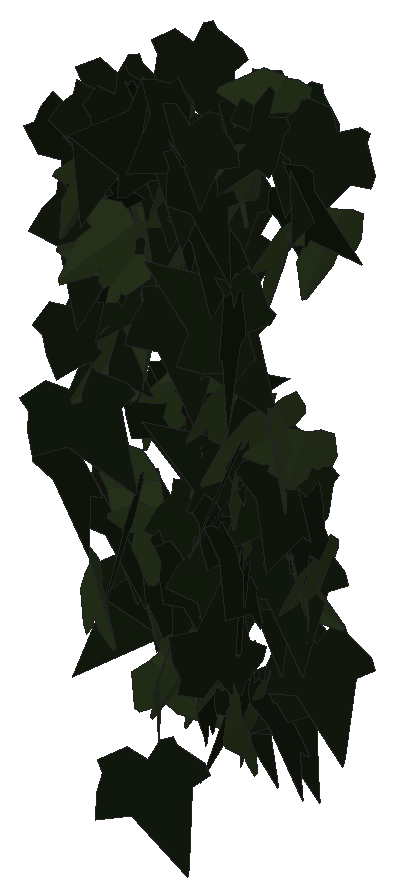
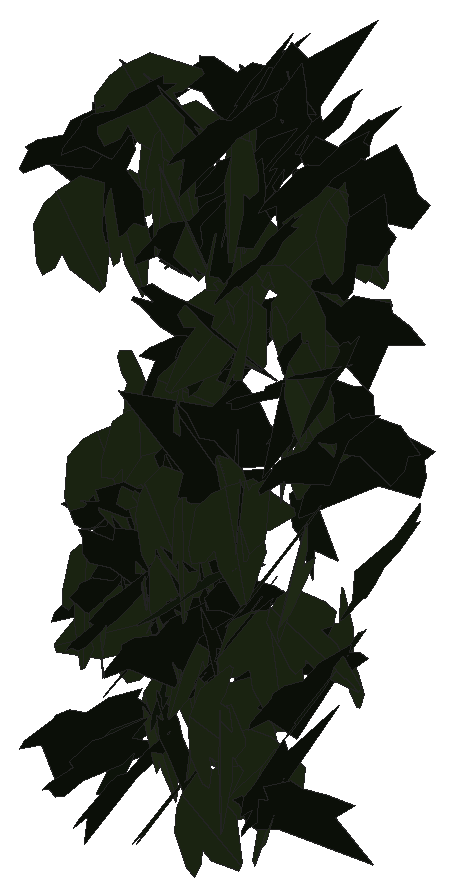
# SketchUp Ruby script. Lengths in inches.
U = 1.inch
M = Sketchup.active_model
def pt(a) = Geom::Point3d.new(a.map { |v| v * U })
def face(e, loops, mat)
  f = e.add_face(loops[0].map { |a| pt(a) })
  loops[1..].each { |l| e.add_face(l.map { |a| pt(a) }).erase! }
  f.material = f.back_material = mat if mat
  f
end
# faces: each face lists its corners as indices into pts; further lists are holes
def faces(e, pts, list, mat = nil) = list.each { |f| face(e, (f[0].is_a?(Array) ? f : [f]).map { |l| l.map { |i| pts[i] } }, mat) }
# xy, xz, yz: faces in a plane at the given z, y or x. An outline is a flat list of corners, or four numbers for a rectangle; further outlines are holes
def ring(l) = l.size == 4 ? [[l[0], l[1]], [l[2], l[1]], [l[2], l[3]], [l[0], l[3]]] : l.each_slice(2).to_a
def flat(e, list, mat, &to3) = list.each { |f| face(e, (f[0].is_a?(Array) ? f : [f]).map { |l| ring(l).map { |u, v| to3.(u, v) } }, mat) }
def xy(e, z, list, mat = nil) = flat(e, list, mat) { |x, y| [x, y, z] }
def xz(e, y, list, mat = nil) = flat(e, list, mat) { |x, z| [x, y, z] }
def yz(e, x, list, mat = nil) = flat(e, list, mat) { |y, z| [x, y, z] }
def lines(e, pts, list) = list.each { |a, b| e.add_line(pt(pts[a]), pt(pts[b])) }
# prism: a flat outline (further loops are holes) pulled along v
def prism(e, loops, v, mat = nil)
  f = face(e, loops, mat); d = Geom::Vector3d.new(v.map { |x| x * U })
  f.pushpull(f.normal.samedirection?(d) ? d.length : -d.length)
end
def box(e, o, s, mat = nil) = prism(e, [[o, [o[0] + s[0], o[1], o[2]], [o[0] + s[0], o[1] + s[1], o[2]], [o[0], o[1] + s[1], o[2]]]], [0, 0, s[2]], mat)
def at(x, y, z, deg = 0) = Geom::Transformation.translation(pt([x, y, z])) * Geom::Transformation.rotation(ORIGIN, Z_AXIS, deg.degrees)
def axes(o, x, y, z) = Geom::Transformation.new([*x, 0, *y, 0, *z, 0, *pt(o).to_a, 1])
def part(name) = M.definitions.add(name)
# library, detail: a bought-in or finely detailed component or shape, given as its bounding box
def library(name, o, s) = part(name).tap { |d| box(d.entities, o, s) }
def detail(e, o, s) = box(e.add_group.entities, o, s)
def put(e, d, t, mat = nil) = e.add_instance(d, t).tap { |i| i.material = mat if mat }
def group(e, t, mat = nil) = e.add_group.tap { |g| g.transformation = t; g.material = mat if mat }.entities
root = M.entities
M.materials.add("efeu1").color = [18, 25, 13]
M.materials.add("efeu2").color = [43, 57, 29]
c1 = part("ivyleaf_9")
p = [[1.54,2.16,1.25],[1.36,2.04,1.19],[-0.21,0.99,0.68],[-0.71,1.11,0.82],[-0.85,0.86,0.67],[-0.8,0.17,0.21],
  [-0.9,-0.01,0.1],[-0.67,-0.16,-0.02],[-0.08,-0.08,-0.05],[-0.03,-0.6,-0.4],[0.65,-0.88,-0.66],[0.83,-0.6,-0.49],
  [1.29,-0.42,-0.43],[1.8125,-0.07,-0.26],[1.21,0.44,0.15]]
faces(c1.entities,p,[[0,1,2,3,4,5,6,7,8,9,10,11,12,13,14]],"efeu1")
c2 = part("ivyleaf_10")
p = [[0,0.5,-0.03],[-0.0625,2.02,-0.43],[-0.19,2.01,-0.46],[-0.54,1.05,-0.29],[-0.52,0.625,-0.18],[-0.83,0.76,-0.28],
  [-1.16,0.64,-0.33],[-1.15,0.33,-0.24],[-0.77,-0.39,0.02],[-0.3,-0.51,0.16],[0.04,-0.48,0.23],[-0.02,2.01,-0.4375],
  [-0.06,2.01,-0.43],[0.04,-0.49,0.23],[0.67,-0.49,0.14],[1.38,0.36,-0.2],[1.375,0.51,-0.24],[0.81,0.65,-0.19],
  [0.62,0.59,-0.15],[0.6,1.09,-0.28],[0.5,1.23,-0.31]]
faces(c2.entities,p,[[0,1,2,3,4,5,6,7,8,9,10],[11,12,0,13,14,15,16,17,18,19,20]],"efeu2")
put(root,c1,axes([30.3,219.35,234.05],[-0.08289,-0.36968,-0.32629],[0.0657,0.31963,-0.37884],[0.48868,-0.10568,-0.00441]))
put(root,c2,axes([29.49,220.625,234.35],[0.06504,-0.16772,-0.46652],[0.15197,-0.44112,0.17978],[-0.47189,-0.16518,-0.00641]))
put(root,c1,axes([30.59,220.63,239.86],[-0.209,0.00128,-0.45422],[0.44781,-0.08313,-0.20629],[-0.07605,-0.49304,0.03361]))
put(root,c1,axes([29.08,220.65,236.79],[-0.26517,0.09797,-0.41242],[0.36855,-0.18705,-0.2814],[-0.20942,-0.45323,0.02698]))
put(root,c1,axes([30.46,220.92,236.13],[-0.00947,-0.27867,0.41503],[0.08144,-0.41042,-0.27372],[0.49323,0.06242,0.05316]))
put(root,c2,axes([30.86,220.47,234.28],[-0.27139,0.1393,0.39616],[-0.37466,0.13274,-0.30333],[-0.18968,-0.46149,0.03233]))
put(root,c1,axes([29.02,221,241.49],[-0.03894,-0.04823,0.49614],[-0.31224,-0.38557,-0.06199],[0.38857,-0.31466,-0.00009]))
put(root,c2,axes([28.22,220.84,235.23],[0.15955,-0.10346,0.46243],[0.43514,-0.16118,-0.1862],[0.1876,0.46186,0.03861]))
put(root,c1,axes([30.46,220.5,234.86],[-0.22152,-0.24857,0.37302],[0.25211,0.27495,0.33293],[-0.37064,0.33558,0.00352]))
put(root,c1,axes([30.5,220.85,235.49],[-0.07678,0.22238,0.44119],[0.04162,-0.44199,0.23003],[0.49231,0.07204,0.04936]))
put(root,c2,axes([28.39,221.12,239.97],[-0.09483,-0.078,0.48469],[0.05375,-0.49233,-0.06871],[0.48797,0.03907,0.10176]))
put(root,c1,axes([28.01,220.73,237.8],[-0.07041,-0.26083,-0.42072],[0.20278,0.37247,-0.26485],[0.45158,-0.20793,0.05334]))
put(root,c1,axes([30.43,221.01,239.42],[-0.30565,-0.35395,-0.1769],[-0.11675,-0.13291,0.46766],[-0.37808,0.32719,-0.0014]))
put(root,c1,axes([27.57,221.12,236.65],[0.16765,-0.44128,0.16482],[0.07238,-0.14874,-0.47184],[0.46546,0.18207,0.01401]))
put(root,c1,axes([29.28,221.33,241.6875],[-0.12302,-0.2623,0.40751],[-0.0729,-0.40563,-0.2831],[0.47911,-0.12907,0.06156]))
put(root,c1,axes([28.11,221.26,241.4],[-0.05061,-0.47144,0.1587],[-0.01167,-0.15835,-0.47412],[0.49729,-0.0517,0.00502]))
put(root,c1,axes([29.5,221.125,241.83],[-0.31625,-0.29552,-0.25031],[0.18545,0.16815,-0.43282],[0.33999,-0.3666,0.00326]))
put(root,c1,axes([29.62,221.16,241.26],[0.19437,-0.46058,-0.00935],[-0.00344,0.0087,-0.49991],[0.46066,0.1944,0.00021]))
put(root,c2,axes([27.96,221.3,240.74],[-0.00888,-0.43711,0.2426],[0.00097,-0.24265,-0.43717],[0.49992,-0.0073,0.00516]))
put(root,c2,axes([30.22,220.85,234.87],[0.00907,-0.34479,-0.36199],[0.01537,0.36207,-0.34448],[0.49968,-0.00487,0.01717]))
put(root,c1,axes([27.6,221.11,240.79],[-0.03188,0.02294,0.49845],[0.45927,-0.19391,0.0383],[0.19507,0.4603,-0.00871]))
put(root,c1,axes([30.03,221.37,235.82],[-0.1785,-0.46206,-0.06811],[0.02124,0.06481,-0.49533],[0.46657,-0.17973,-0.00351]))
put(root,c1,axes([28.61,221.47,241.41],[0.10847,-0.18642,0.45109],[0.23745,-0.38357,-0.21561],[0.42644,0.261,0.00532]))
put(root,c1,axes([27.72,221.41,240.39],[0.0658,-0.19236,0.4568],[0.34538,-0.31272,-0.18144],[0.3555,0.33942,0.09172]))
put(root,c2,axes([28.18,221.57,238.15],[0.04719,0.20002,-0.45581],[-0.14564,-0.43227,-0.20477],[-0.47599,0.15209,0.01747]))
put(root,c2,axes([29.27,221.56,234.39],[0.04042,-0.3632,0.34125],[0.03696,-0.33924,-0.36544],[0.49699,0.05477,-0.00058]))
put(root,c1,axes([29.85,221.06,233.82],[0.00612,-0.05402,0.49704],[-0.12932,0.47999,0.05376],[-0.48295,-0.12921,-0.0081]))
put(root,c1,axes([29.23,221.4375,239.13],[-0.09843,-0.46169,-0.16477],[0.0218,0.16377,-0.47191],[0.48973,-0.10009,-0.01212]))
put(root,c1,axes([29.5,221.64,240.25],[0.02345,-0.43904,0.2381],[0.08035,-0.23194,-0.4356],[0.49294,0.0587,0.05967]))
put(root,c1,axes([28.26,221.3,241.75],[0.2348,-0.36099,-0.25408],[-0.08527,0.24528,-0.42728],[0.43313,0.24398,0.05362]))
put(root,c2,axes([30.55,221.5,237.86],[-0.29786,0.28165,-0.28627],[0.14146,-0.25999,-0.40298],[-0.37586,-0.32105,0.0752]))
put(root,c1,axes([27.55,221.35,238.53],[0.01705,-0.1699,-0.46994],[0.38013,0.30962,-0.09815],[0.32436,-0.35393,0.13973]))
put(root,c1,axes([29.1875,221.47,235.54],[0.24265,-0.43319,-0.05885],[-0.0354,0.04762,-0.49647],[0.43574,0.2451,-0.00756]))
put(root,c1,axes([29.93,221.53,237.3125],[-0.29872,0.23806,-0.32264],[0.25552,-0.19703,-0.38196],[-0.30899,-0.39307,-0.00395]))
put(root,c2,axes([28.24,221.69,239.4],[-0.08156,-0.06123,-0.48949],[-0.36598,-0.32515,0.10165],[-0.33076,0.37487,0.00822]))
put(root,c2,axes([30.31,221.5,234.1],[0.20598,-0.45349,0.04383],[0.01724,-0.04031,-0.49807],[0.45527,0.2067,-0.00098]))
put(root,c1,axes([27.72,221.59,239.87],[-0.35755,-0.28123,-0.20754],[0.1589,0.13365,-0.45485],[0.31131,-0.39121,-0.0062]))
put(root,c1,axes([30.38,221.71,233.84],[0.18321,-0.39454,0.24652],[0.10818,-0.22156,-0.43498],[0.45247,0.21272,0.00418]))
put(root,c1,axes([29.27,221.83,238.8125],[-0.08752,-0.25287,0.42237],[0.15927,-0.42047,-0.21873],[0.4658,0.09625,0.15415]))
put(root,c2,axes([29.37,221.34,240.68],[-0.36763,0.30569,0.14629],[-0.10957,0.09703,-0.4781],[-0.32069,-0.38359,-0.00436]))
put(root,c1,axes([30.42,221.87,236.8],[-0.04683,-0.41229,0.27897],[0.07073,-0.28287,-0.40618],[0.49275,0.00142,0.08481]))
put(root,c1,axes([28.84,221.7,241.33],[-0.10901,-0.48029,-0.08627],[0.01411,0.08526,-0.49248],[0.48777,-0.10981,-0.00503]))
put(root,c2,axes([28.02,221.31,240.7],[-0.26382,-0.22076,-0.36285],[0.27723,0.23411,-0.344],[0.32178,-0.3827,-0.00112]))
put(root,c2,axes([29.76,221.45,238.1],[0.02352,-0.47181,-0.16383],[0.00743,0.16433,-0.47217],[0.49939,0.01977,0.01474]))
put(root,c2,axes([28.92,221.41,233.96],[-0.33995,-0.1681,-0.32585],[0.31483,0.09393,-0.3769],[0.18793,-0.46143,0.04198]))
put(root,c2,axes([29.09,221.4,241.16],[0.09349,-0.42682,-0.24307],[-0.02596,0.24279,-0.43632],[0.4905,0.0942,0.02324]))
put(root,c1,axes([29.8,221.63,236.61],[-0.30586,0.31264,-0.24229],[0.12387,-0.21515,-0.43401],[-0.37564,-0.32552,0.05416]))
put(root,c1,axes([29.06,221.91,235.45],[-0.01718,-0.44238,0.23239],[-0.02016,-0.23173,-0.4426],[0.4993,-0.02458,-0.00988]))
put(root,c1,axes([30,221.67,234.12],[-0.37969,0.18943,-0.26448],[0.2403,-0.11071,-0.42426],[-0.21929,-0.44929,-0.00697]))
put(root,c2,axes([29.71,221.82,238.28],[-0.13046,-0.06107,0.4788],[-0.36648,-0.31024,-0.13943],[0.31412,-0.38732,0.03619]))
put(root,c1,axes([29.85,221.76,236.72],[-0.01488,0.0085,0.49971],[-0.49927,0.02223,-0.01524],[-0.02248,-0.49943,0.00782]))
put(root,c1,axes([29.62,221.625,236.38],[0.25229,-0.35279,-0.24877],[-0.14533,0.20191,-0.43372],[0.40648,0.29115,-0.00067]))
put(root,c2,axes([29.82,221.76,241.28],[-0.14425,-0.47373,0.0691],[-0.01559,-0.06749,-0.49518],[0.47849,-0.14501,0.0047]))
put(root,c1,axes([29.45,221.63,238.91],[0.06775,-0.36416,-0.33585],[0.08909,0.34241,-0.3533],[0.48731,-0.01197,0.11128]))
put(root,c1,axes([30.1,221.875,241.85],[-0.48847,0.03084,-0.1022],[0.09978,-0.03828,-0.48845],[-0.03795,-0.49758,0.03125]))
put(root,c1,axes([28.51,222.03,240.41],[-0.00432,-0.48282,0.12987],[-0.01025,-0.12977,-0.48276],[0.49988,-0.00683,-0.00877]))
put(root,c1,axes([29.29,221.94,236.09],[-0.21428,0.07322,-0.44578],[0.41423,-0.16505,-0.22622],[-0.18028,-0.46626,0.01007]))
put(root,c2,axes([28.6,221.74,235.74],[-0.44796,-0.18198,0.12734],[-0.11792,-0.04806,-0.48351],[0.18822,-0.46322,0.00014]))
put(root,c1,axes([29.22,221.98,236.05],[-0.20181,-0.45055,-0.07919],[0.02518,0.07548,-0.49363],[0.45677,-0.20323,-0.00778]))
put(root,c1,axes([27.83,221.86,241.64],[0.09223,-0.46529,-0.15811],[-0.00308,0.16032,-0.47359],[0.49141,0.08833,0.02671]))
put(root,c1,axes([29.4,221.91,237.86],[-0.23489,-0.12463,-0.42343],[0.40536,0.12891,-0.26281],[0.17468,-0.46674,0.04048]))
put(root,c1,axes([29.12,221.58,240.5],[0.18626,-0.1046,-0.45207],[-0.37646,0.25072,-0.21312],[0.27127,0.41976,0.01464]))
put(root,c2,axes([28.89,221.82,240.34],[-0.09418,-0.487,-0.06292],[0.01123,0.06191,-0.49603],[0.49092,-0.09484,-0.00072]))
put(root,c1,axes([28.91,222,237.09],[-0.18251,0.18695,0.42631],[0.02636,-0.45302,0.20995],[0.46475,0.09911,0.1555]))
put(root,c2,axes([28.47,221.59,238.37],[0.17955,-0.23286,-0.4044],[-0.13524,0.38874,-0.28389],[0.44662,0.21133,0.07661]))
put(root,c2,axes([30.375,221.94,240.31],[0.10822,-0.48555,0.05034],[0.01308,-0.04866,-0.49745],[0.48797,0.10898,0.00217]))
put(root,c1,axes([27.59,221.99,235.69],[0.2269,-0.44524,0.01669],[-0.001,-0.01924,-0.49963],[0.44555,0.22669,-0.00962]))
put(root,c1,axes([28.97,221.79,237.68],[0.0985,-0.03755,0.48876],[0.47664,-0.10913,-0.10444],[0.11452,0.4865,0.0143]))
put(root,c1,axes([30.44,222.01,235.84],[-0.07736,-0.47145,-0.14749],[0.01536,0.14692,-0.47768],[0.49374,-0.07844,-0.00824]))
put(root,c2,axes([29.86,221.9,235.96],[0.17049,-0.46485,-0.06962],[-0.02613,0.06457,-0.49512],[0.46931,0.17246,-0.00227]))
put(root,c2,axes([27.96,222,240.06],[-0.38927,0.08537,-0.30197],[0.23703,-0.23531,-0.37208],[-0.20564,-0.43283,0.14273]))
put(root,c1,axes([29.71,221.79,236.63],[-0.04987,-0.09963,-0.48743],[0.31165,0.37559,-0.10866],[0.3878,-0.31465,0.02464]))
put(root,c2,axes([28.16,221.89,236.12],[0.24018,-0.08445,-0.43033],[-0.41299,0.12146,-0.25434],[0.14749,0.47761,-0.01141]))
put(root,c1,axes([28.15,222.3,239.07],[-0.30404,-0.36278,0.16108],[0.01506,-0.2133,-0.45197],[0.39665,-0.26999,0.14063]))
put(root,c1,axes([27.7,222.21,238.47],[-0.07892,-0.49117,0.05025],[-0.00825,-0.04957,-0.49747],[0.49366,-0.07935,-0.00028]))
put(root,c2,axes([29.95,221.65,236.88],[-0.00104,0.34583,0.36111],[-0.23645,0.31784,-0.30507],[-0.44056,-0.1714,0.16288]))
put(root,c2,axes([30.13,221.9375,237.7],[-0.14215,-0.4746,-0.06745],[0.00974,0.06748,-0.49533],[0.47927,-0.14213,-0.00994]))
put(root,c2,axes([29.85,221.84,237.22],[-0.22157,-0.40419,-0.19375],[0.07853,0.17778,-0.46068],[0.44129,-0.23457,-0.0153]))
put(root,c2,axes([29.47,222.15,236.53],[-0.07948,-0.46053,0.17775],[0.0782,-0.18951,-0.45604],[0.48741,-0.04469,0.10216]))
put(root,c2,axes([30.5,222.08,237.37],[-0.22836,-0.42242,0.13934],[-0.05049,-0.131,-0.47988],[0.44193,-0.23324,0.01717]))
put(root,c1,axes([29.82,222.1875,235.4375],[0.13839,-0.47543,0.06935],[0.01718,-0.06723,-0.49516],[0.48016,0.13944,-0.00227]))
put(root,c1,axes([30.36,222.27,236.94],[-0.41608,-0.26384,0.08524],[-0.0537,-0.07412,-0.49155],[0.27202,-0.4182,0.03334]))
put(root,c1,axes([29.47,222.09,233.8125],[0.24286,-0.43505,-0.04183],[-0.01731,0.03825,-0.49823],[0.43671,0.24345,0.00352]))
put(root,c1,axes([30.85,221.76,236.17],[-0.0474,0.06684,0.49324],[-0.23427,0.43416,-0.08135],[-0.43917,-0.23882,-0.00984]))
put(root,c1,axes([30.29,222.06,240.84],[0.13339,-0.03096,-0.48088],[0.45777,0.16401,0.11642],[0.15053,-0.47132,0.0721]))
put(root,c2,axes([28.33,221.97,234.14],[-0.32005,0.3806,-0.05207],[0.02989,-0.0429,-0.49726],[-0.38298,-0.32141,0.00471]))
put(root,c1,axes([29.24,222.22,240.66],[-0.05119,-0.49356,-0.06147],[0.01149,0.0606,-0.49618],[0.49724,-0.05221,0.00514]))
put(root,c2,axes([27.78,222.21,239.25],[0.13275,-0.44651,0.18169],[0.04319,-0.17667,-0.46575],[0.48012,0.13935,-0.00833]))
put(root,c1,axes([27.53,222.1,239.21],[0.31287,-0.39001,-0.00086],[-0.0005,0.0007,-0.5],[0.39001,0.31288,0.00005]))
put(root,c2,axes([30.29,221.83,236.58],[0.16601,-0.26622,-0.38931],[-0.19976,0.33419,-0.31371],[0.42724,0.2597,0.0046]))
put(root,c1,axes([28.6,222.29,240.67],[0.06462,-0.21206,0.44817],[0.27101,-0.36336,-0.211],[0.41518,0.27019,0.06798]))
put(root,c2,axes([30.8125,221.96,235.85],[0.00874,-0.4652,-0.18306],[-0.00932,0.18291,-0.46525],[0.49984,0.01155,-0.00547]))
put(root,c1,axes([28.01,221.72,239.24],[-0.004,-0.01008,-0.49988],[-0.34002,0.36655,-0.00467],[0.36656,0.33991,-0.00979]))
put(root,c2,axes([29.97,222.26,242.02],[-0.25583,-0.35789,0.23762],[-0.06003,-0.24406,-0.43224],[0.42538,-0.24969,0.08191]))
put(root,c2,axes([30.78,221.76,235.33],[0.02637,0.04509,-0.49726],[-0.21734,0.44934,0.02922],[0.44952,0.21461,0.0433]))
put(root,c2,axes([30.16,222,235.43],[0.22641,-0.06702,0.44074],[0.41748,0.20526,-0.18325],[-0.15637,0.45098,0.1489]))
put(root,c1,axes([27.69,222.29,235.74],[-0.00015,-0.49706,-0.05415],[-0.00776,0.05415,-0.497],[0.49994,0.00069,-0.00773]))
put(root,c2,axes([29.75,221.98,241.16],[0.04924,-0.4359,-0.23993],[-0.01379,0.23981,-0.43852],[0.49738,0.0498,0.01159]))
put(root,c1,axes([28.14,222.51,234.24],[-0.12336,-0.07418,0.47883],[-0.18318,-0.4503,-0.11695],[0.44858,-0.20428,0.08392]))
put(root,c1,axes([30.09,222.24,233.78],[0.1639,-0.4593,-0.11039],[-0.03108,0.10611,-0.48762],[0.47135,0.1667,0.00623]))
put(root,c2,axes([29,222.43,233.82],[0.0467,-0.41031,0.28189],[0.04042,-0.27906,-0.4129],[0.49617,0.06135,0.0071]))
put(root,c2,axes([28.46,222.29,237.28],[-0.30697,0.0797,0.38655],[0.37814,-0.08087,0.31697],[0.11305,0.48694,-0.01062]))
put(root,c1,axes([27.96,222.45,234.29],[-0.4498,-0.20882,0.06381],[-0.05592,-0.03109,-0.49589],[0.21107,-0.45324,0.00461]))
put(root,c1,axes([27.97,222.25,237.17],[0.27427,-0.4044,-0.10601],[-0.04648,0.0965,-0.48839],[0.41547,0.27775,0.01534]))
put(root,c1,axes([30.15,222.65,235.76],[-0.18024,-0.30749,0.35066],[-0.0908,-0.34561,-0.34973],[0.45746,-0.18975,0.06875]))
put(root,c2,axes([28.78,222.05,241.43],[0.35252,-0.21275,-0.28368],[-0.08935,0.33381,-0.36137],[0.34315,0.30547,0.19733]))
put(root,c2,axes([29.08,222.4,240.46],[0.26821,-0.22641,-0.3561],[0.28405,-0.21516,0.35074],[-0.31206,-0.39044,0.01321]))
put(root,c2,axes([30.71,222.45,240.34],[-0.13245,-0.43927,0.19875],[-0.00985,-0.2036,-0.45656],[0.48204,-0.12486,0.04528]))
put(root,c1,axes([30.5,222.39,234.41],[-0.02302,-0.46684,-0.17757],[0.05982,0.1739,-0.46495],[0.49588,-0.04265,0.04784]))
put(root,c1,axes([30.36,222.7,233.99],[-0.231,-0.33521,0.2903],[-0.10753,-0.27522,-0.40335],[0.4302,-0.24878,0.05506]))
put(root,c2,axes([29.31,222.22,237.04],[0.11889,-0.44951,-0.18387],[-0.01704,0.18532,-0.46408],[0.48536,0.11661,0.02875]))
put(root,c1,axes([30,222.52,241.84],[-0.0702,-0.4935,-0.03911],[0.0003,0.03946,-0.49844],[0.49505,-0.07001,-0.00524]))
put(root,c2,axes([29.51,222.46,237.29],[0.07595,-0.47824,0.12458],[0.01515,-0.12373,-0.48421],[0.49397,0.07733,-0.0043]))
put(root,c2,axes([28.77,222.26,234.72],[0.20487,-0.43646,-0.13241],[0.02445,0.15546,-0.47459],[0.45544,0.18799,0.08504]))
put(root,c2,axes([27.67,222.57,236.76],[-0.25925,0.13828,0.40456],[0.26784,-0.31625,0.27973],[0.33324,0.36175,0.0899]))
put(root,c2,axes([29.2,222.04,234.92],[0.04329,-0.23939,-0.43683],[-0.09937,0.42551,-0.24303],[0.48811,0.10786,-0.01073]))
put(root,c1,axes([28.61,222.37,242.125],[0.11283,-0.44799,-0.19124],[0.00321,0.19698,-0.45955],[0.48709,0.10247,0.04733]))
put(root,c2,axes([28.59,222.39,237.5],[-0.1876,-0.46044,0.05292],[-0.00863,-0.05361,-0.49704],[0.46339,-0.1874,0.01217]))
put(root,c1,axes([29.98,222.52,236.6875],[-0.46119,-0.17899,-0.07256],[0.06369,0.03639,-0.49459],[0.18233,-0.46545,-0.01077]))
put(root,c2,axes([28.73,222.67,235.04],[0.09292,-0.30534,0.38488],[0.19555,-0.33635,-0.31405],[0.4507,0.20889,0.05691]))
put(root,c1,axes([29.43,222.51,239.72],[-0.48145,0.02657,0.13228],[-0.13345,-0.02151,-0.48138],[-0.01989,-0.49883,0.0278]))
put(root,c1,axes([29.37,222.6,235.84],[-0.10952,-0.48687,-0.03099],[0.00379,0.03091,-0.49903],[0.48784,-0.10954,-0.00308]))
put(root,c2,axes([28.33,222.46,239.83],[-0.18074,0.4102,-0.22152],[0.06753,-0.21205,-0.44775],[-0.46127,-0.19177,0.02125]))
put(root,c1,axes([30.54,222.67,241.43],[-0.21256,-0.44856,0.06011],[-0.01982,-0.05712,-0.49633],[0.45213,-0.21338,0.0065]))
put(root,c1,axes([28.86,222.71,236.5625],[-0.05396,-0.47591,0.14353],[0.1362,-0.153,-0.45611],[0.47805,-0.01013,0.14615]))
put(root,c2,axes([28.76,222.17,239.71],[-0.18968,-0.29652,-0.3551],[0.19287,0.29816,-0.35199],[0.4205,-0.27051,0.00127]))
